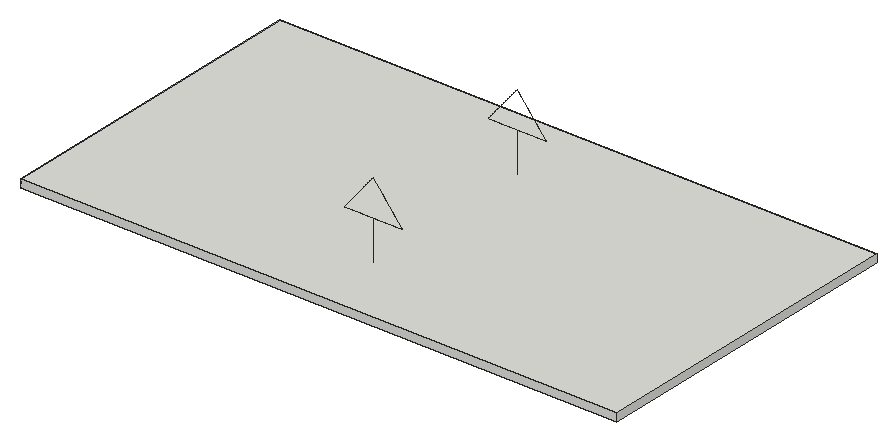
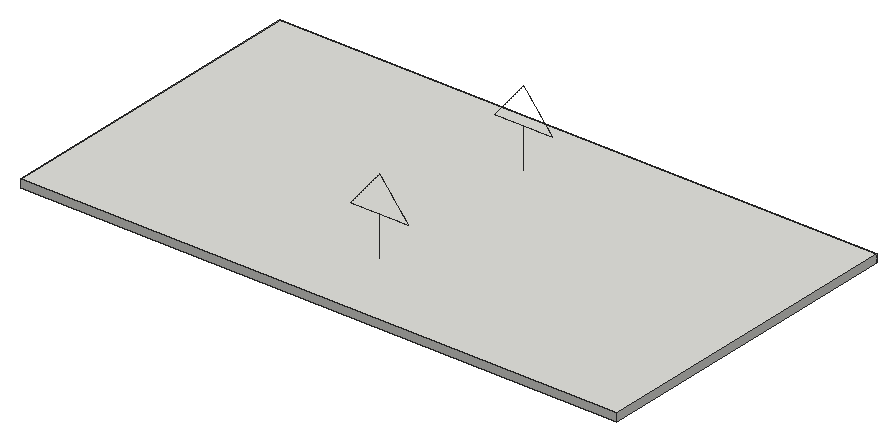
# SketchUp Ruby script. Lengths in inches.
U = 1.inch
M = Sketchup.active_model
def pt(a) = Geom::Point3d.new(a.map { |v| v * U })
def face(e, loops, mat)
  f = e.add_face(loops[0].map { |a| pt(a) })
  loops[1..].each { |l| e.add_face(l.map { |a| pt(a) }).erase! }
  f.material = f.back_material = mat if mat
  f
end
# faces: each face lists its corners as indices into pts; further lists are holes
def faces(e, pts, list, mat = nil) = list.each { |f| face(e, (f[0].is_a?(Array) ? f : [f]).map { |l| l.map { |i| pts[i] } }, mat) }
# xy, xz, yz: faces in a plane at the given z, y or x. An outline is a flat list of corners, or four numbers for a rectangle; further outlines are holes
def ring(l) = l.size == 4 ? [[l[0], l[1]], [l[2], l[1]], [l[2], l[3]], [l[0], l[3]]] : l.each_slice(2).to_a
def flat(e, list, mat, &to3) = list.each { |f| face(e, (f[0].is_a?(Array) ? f : [f]).map { |l| ring(l).map { |u, v| to3.(u, v) } }, mat) }
def xy(e, z, list, mat = nil) = flat(e, list, mat) { |x, y| [x, y, z] }
def xz(e, y, list, mat = nil) = flat(e, list, mat) { |x, z| [x, y, z] }
def yz(e, x, list, mat = nil) = flat(e, list, mat) { |y, z| [x, y, z] }
def lines(e, pts, list) = list.each { |a, b| e.add_line(pt(pts[a]), pt(pts[b])) }
# prism: a flat outline (further loops are holes) pulled along v
def prism(e, loops, v, mat = nil)
  f = face(e, loops, mat); d = Geom::Vector3d.new(v.map { |x| x * U })
  f.pushpull(f.normal.samedirection?(d) ? d.length : -d.length)
end
def box(e, o, s, mat = nil) = prism(e, [[o, [o[0] + s[0], o[1], o[2]], [o[0] + s[0], o[1] + s[1], o[2]], [o[0], o[1] + s[1], o[2]]]], [0, 0, s[2]], mat)
def at(x, y, z, deg = 0) = Geom::Transformation.translation(pt([x, y, z])) * Geom::Transformation.rotation(ORIGIN, Z_AXIS, deg.degrees)
def axes(o, x, y, z) = Geom::Transformation.new([*x, 0, *y, 0, *z, 0, *pt(o).to_a, 1])
def part(name) = M.definitions.add(name)
# library, detail: a bought-in or finely detailed component or shape, given as its bounding box
def library(name, o, s) = part(name).tap { |d| box(d.entities, o, s) }
def detail(e, o, s) = box(e.add_group.entities, o, s)
def put(e, d, t, mat = nil) = e.add_instance(d, t).tap { |i| i.material = mat if mat }
def group(e, t, mat = nil) = e.add_group.tap { |g| g.transformation = t; g.material = mat if mat }.entities
root = M.entities
c1 = part("Group84\#1")
p = [[0,0,0],[0,0,-43.36],[-21.49,0,-43.36],[139.88,-0.5,0],[-139.88,-0.5,0],[139.88,0.5,0],
  [139.88,0,0],[-139.88,0.5,0],[21.49,0,-43.36],[-139.88,0,0],[0,0,-70.19]]
lines(c1.entities,p,[[0,1],[1,2],[3,4],[5,6],[7,5],[1,8],[9,0],[0,6],[8,10],[4,9],[6,3],[2,10],
  [9,7]])
c2 = part("Rectangle Light")
put(c2.entities,c1,at(0,0,0))
c3 = part("Group")
box(c3.entities,[0,0,0],[440.75,240,6])
xy(root,232,[[[79.99,50,360.75,184],[80.99,51,359.75,183]]])
xy(root,233,[[[80.99,51,359.75,183],[81.99,52,358.75,182]]])
xy(root,234,[[[57.99,28,382.75,206],[79.99,50,360.75,184],[370.5625,111,370.19,111.03,369.8125,111.07,369.44,111.14,369.08,111.24,368.72,111.35,368.37,111.49,368.03,111.65,367.7,111.84,367.38,112.04,367.07,112.26,366.78,112.5,366.51,112.76,366.25,113.03,366.01,113.32,365.79,113.63,365.59,113.95,365.4,114.28,365.24,114.62,365.1,114.97,364.99,115.33,364.89,115.69,364.82,116.0625,364.78,116.44,364.75,116.8125,364.75,117.1875,364.78,117.56,364.82,117.9375,364.89,118.31,364.99,118.67,365.1,119.03,365.24,119.38,365.4,119.72,365.59,120.05,365.79,120.37,366.01,120.68,366.25,120.97,366.51,121.24,366.78,121.5,367.07,121.74,367.38,121.96,367.7,122.16,368.03,122.35,368.37,122.51,368.72,122.65,369.08,122.76,369.44,122.86,369.8125,122.93,370.19,122.97,370.5625,123,370.9375,123,371.31,122.97,371.6875,122.93,372.06,122.86,372.42,122.76,372.78,122.65,373.13,122.51,373.47,122.35,373.8,122.16,374.12,121.96,374.43,121.74,374.72,121.5,374.99,121.24,375.25,120.97,375.49,120.68,375.71,120.37,375.91,120.05,376.1,119.72,376.26,119.38,376.4,119.03,376.51,118.67,376.61,118.31,376.68,117.9375,376.72,117.56,376.75,117.1875,376.75,116.8125,376.72,116.44,376.68,116.0625,376.61,115.69,376.51,115.33,376.4,114.97,376.26,114.62,376.1,114.28,375.91,113.95,375.71,113.63,375.49,113.32,375.25,113.03,374.99,112.76,374.72,112.5,374.43,112.26,374.12,112.04,373.8,111.84,373.47,111.65,373.13,111.49,372.78,111.35,372.42,111.24,372.06,111.14,371.6875,111.07,371.31,111.03,370.9375,111],[220.18,34,219.81,34.03,219.43,34.07,219.0625,34.14,218.7,34.24,218.34,34.35,217.99,34.49,217.65,34.65,217.32,34.84,217,35.04,216.69,35.26,216.4,35.5,216.13,35.76,215.87,36.03,215.63,36.32,215.41,36.63,215.21,36.95,215.02,37.28,214.86,37.62,214.73,37.97,214.61,38.33,214.52,38.69,214.44,39.0625,214.4,39.44,214.375,39.8125,214.375,40.1875,214.4,40.56,214.44,40.9375,214.52,41.31,214.61,41.67,214.73,42.03,214.86,42.38,215.02,42.72,215.21,43.05,215.41,43.37,215.63,43.68,215.87,43.97,216.13,44.24,216.4,44.5,216.69,44.74,217,44.96,217.32,45.16,217.65,45.35,217.99,45.51,218.34,45.65,218.7,45.76,219.0625,45.86,219.43,45.93,219.81,45.97,220.18,46,220.56,46,220.94,45.97,221.31,45.93,221.68,45.86,222.04,45.76,222.4,45.65,222.75,45.51,223.09,45.35,223.43,45.16,223.74,44.96,224.05,44.74,224.34,44.5,224.61,44.24,224.87,43.97,225.11,43.68,225.33,43.37,225.54,43.05,225.72,42.72,225.88,42.38,226.02,42.03,226.13,41.67,226.23,41.31,226.3,40.9375,226.34,40.56,226.37,40.1875,226.37,39.8125,226.34,39.44,226.3,39.0625,226.23,38.69,226.13,38.33,226.02,37.97,225.88,37.62,225.72,37.28,225.54,36.95,225.33,36.63,225.11,36.32,224.87,36.03,224.61,35.76,224.34,35.5,224.05,35.26,223.74,35.04,223.43,34.84,223.09,34.65,222.75,34.49,222.4,34.35,222.04,34.24,221.68,34.14,221.31,34.07,220.94,34.03,220.56,34],[295.37,34,295,34.03,294.62,34.07,294.25,34.14,293.89,34.24,293.53,34.35,293.18,34.49,292.84,34.65,292.51,34.84,292.1875,35.04,291.88,35.26,291.59,35.5,291.32,35.76,291.06,36.03,290.82,36.32,290.6,36.63,290.4,36.95,290.21,37.28,290.05,37.62,289.92,37.97,289.8,38.33,289.7,38.69,289.63,39.0625,289.59,39.44,289.5625,39.8125,289.5625,40.1875,289.59,40.56,289.63,40.9375,289.7,41.31,289.8,41.67,289.92,42.03,290.05,42.38,290.21,42.72,290.4,43.05,290.6,43.37,290.82,43.68,291.06,43.97,291.32,44.24,291.59,44.5,291.88,44.74,292.1875,44.96,292.51,45.16,292.84,45.35,293.18,45.51,293.53,45.65,293.89,45.76,294.25,45.86,294.62,45.93,295,45.97,295.37,46,295.75,46,296.125,45.97,296.5,45.93,296.87,45.86,297.23,45.76,297.59,45.65,297.94,45.51,298.28,45.35,298.61,45.16,298.93,44.96,299.24,44.74,299.53,44.5,299.8,44.24,300.0625,43.97,300.3,43.68,300.52,43.37,300.72,43.05,300.91,42.72,301.07,42.38,301.21,42.03,301.32,41.67,301.42,41.31,301.49,40.9375,301.53,40.56,301.56,40.1875,301.56,39.8125,301.53,39.44,301.49,39.0625,301.42,38.69,301.32,38.33,301.21,37.97,301.07,37.62,300.91,37.28,300.72,36.95,300.52,36.63,300.3,36.32,300.0625,36.03,299.8,35.76,299.53,35.5,299.24,35.26,298.93,35.04,298.61,34.84,298.28,34.65,297.94,34.49,297.59,34.35,297.23,34.24,296.87,34.14,296.5,34.07,296.125,34.03,295.75,34],[370.5625,34,370.19,34.03,369.8125,34.07,369.44,34.14,369.08,34.24,368.72,34.35,368.37,34.49,368.03,34.65,367.7,34.84,367.38,35.04,367.07,35.26,366.78,35.5,366.51,35.76,366.25,36.03,366.01,36.32,365.79,36.63,365.59,36.95,365.4,37.28,365.24,37.62,365.1,37.97,364.99,38.33,364.89,38.69,364.82,39.0625,364.78,39.44,364.75,39.8125,364.75,40.1875,364.78,40.56,364.82,40.9375,364.89,41.31,364.99,41.67,365.1,42.03,365.24,42.38,365.4,42.72,365.59,43.05,365.79,43.37,366.01,43.68,366.25,43.97,366.51,44.24,366.78,44.5,367.07,44.74,367.38,44.96,367.7,45.16,368.03,45.35,368.37,45.51,368.72,45.65,369.08,45.76,369.44,45.86,369.8125,45.93,370.19,45.97,370.5625,46,370.9375,46,371.31,45.97,371.6875,45.93,372.06,45.86,372.42,45.76,372.78,45.65,373.13,45.51,373.47,45.35,373.8,45.16,374.12,44.96,374.43,44.74,374.72,44.5,374.99,44.24,375.25,43.97,375.49,43.68,375.71,43.37,375.91,43.05,376.1,42.72,376.26,42.38,376.4,42.03,376.51,41.67,376.61,41.31,376.68,40.9375,376.72,40.56,376.75,40.1875,376.75,39.8125,376.72,39.44,376.68,39.0625,376.61,38.69,376.51,38.33,376.4,37.97,376.26,37.62,376.1,37.28,375.91,36.95,375.71,36.63,375.49,36.32,375.25,36.03,374.99,35.76,374.72,35.5,374.43,35.26,374.12,35.04,373.8,34.84,373.47,34.65,373.13,34.49,372.78,34.35,372.42,34.24,372.06,34.14,371.6875,34.07,371.31,34.03,370.9375,34],[144.99,188,144.62,188.03,144.24,188.07,143.87,188.14,143.51,188.24,143.15,188.35,142.8,188.49,142.46,188.65,142.125,188.84,141.81,189.04,141.5,189.26,141.21,189.5,140.9375,189.76,140.68,190.03,140.44,190.32,140.22,190.63,140.02,190.95,139.84,191.28,139.67,191.62,139.54,191.97,139.42,192.33,139.33,192.69,139.26,193.0625,139.21,193.44,139.18,193.8125,139.18,194.1875,139.21,194.56,139.26,194.9375,139.33,195.31,139.42,195.67,139.54,196.03,139.67,196.38,139.84,196.72,140.02,197.05,140.22,197.37,140.44,197.68,140.68,197.97,140.9375,198.24,141.21,198.5,141.5,198.74,141.81,198.96,142.125,199.16,142.46,199.35,142.8,199.51,143.15,199.65,143.51,199.76,143.87,199.86,144.24,199.93,144.62,199.97,144.99,200,145.37,200,145.75,199.97,146.12,199.93,146.49,199.86,146.86,199.76,147.21,199.65,147.5625,199.51,147.91,199.35,148.24,199.16,148.55,198.96,148.86,198.74,149.15,198.5,149.42,198.24,149.68,197.97,149.92,197.68,150.14,197.37,150.35,197.05,150.53,196.72,150.6875,196.38,150.83,196.03,150.94,195.67,151.04,195.31,151.11,194.9375,151.15,194.56,151.18,194.1875,151.18,193.8125,151.15,193.44,151.11,193.0625,151.04,192.69,150.94,192.33,150.83,191.97,150.6875,191.62,150.53,191.28,150.35,190.95,150.14,190.63,149.92,190.32,149.68,190.03,149.42,189.76,149.15,189.5,148.86,189.26,148.55,189.04,148.24,188.84,147.91,188.65,147.5625,188.49,147.21,188.35,146.86,188.24,146.49,188.14,146.12,188.07,145.75,188.03,145.37,188],[69.8,188,69.43,188.03,69.05,188.07,68.68,188.14,68.32,188.24,67.96,188.35,67.61,188.49,67.27,188.65,66.9375,188.84,66.62,189.04,66.3125,189.26,66.02,189.5,65.75,189.76,65.49,190.03,65.25,190.32,65.03,190.63,64.83,190.95,64.65,191.28,64.48,191.62,64.35,191.97,64.23,192.33,64.14,192.69,64.07,193.0625,64.02,193.44,63.99,193.8125,63.99,194.1875,64.02,194.56,64.07,194.9375,64.14,195.31,64.23,195.67,64.35,196.03,64.48,196.38,64.65,196.72,64.83,197.05,65.03,197.37,65.25,197.68,65.49,197.97,65.75,198.24,66.02,198.5,66.3125,198.74,66.62,198.96,66.9375,199.16,67.27,199.35,67.61,199.51,67.96,199.65,68.32,199.76,68.68,199.86,69.05,199.93,69.43,199.97,69.8,200,70.18,200,70.56,199.97,70.93,199.93,71.3,199.86,71.67,199.76,72.02,199.65,72.375,199.51,72.72,199.35,73.05,199.16,73.36,198.96,73.67,198.74,73.96,198.5,74.23,198.24,74.49,197.97,74.73,197.68,74.95,197.37,75.16,197.05,75.34,196.72,75.5,196.38,75.64,196.03,75.75,195.67,75.85,195.31,75.92,194.9375,75.96,194.56,75.99,194.1875,75.99,193.8125,75.96,193.44,75.92,193.0625,75.85,192.69,75.75,192.33,75.64,191.97,75.5,191.62,75.34,191.28,75.16,190.95,74.95,190.63,74.73,190.32,74.49,190.03,74.23,189.76,73.96,189.5,73.67,189.26,73.36,189.04,73.05,188.84,72.72,188.65,72.375,188.49,72.02,188.35,71.67,188.24,71.3,188.14,70.93,188.07,70.56,188.03,70.18,188],[69.8,111,69.43,111.03,69.05,111.07,68.68,111.14,68.32,111.24,67.96,111.35,67.61,111.49,67.27,111.65,66.9375,111.84,66.62,112.04,66.3125,112.26,66.02,112.5,65.75,112.76,65.49,113.03,65.25,113.32,65.03,113.63,64.83,113.95,64.65,114.28,64.48,114.62,64.35,114.97,64.23,115.33,64.14,115.69,64.07,116.0625,64.02,116.44,63.99,116.8125,63.99,117.1875,64.02,117.56,64.07,117.9375,64.14,118.31,64.23,118.67,64.35,119.03,64.48,119.38,64.65,119.72,64.83,120.05,65.03,120.37,65.25,120.68,65.49,120.97,65.75,121.24,66.02,121.5,66.3125,121.74,66.62,121.96,66.9375,122.16,67.27,122.35,67.61,122.51,67.96,122.65,68.32,122.76,68.68,122.86,69.05,122.93,69.43,122.97,69.8,123,70.18,123,70.56,122.97,70.93,122.93,71.3,122.86,71.67,122.76,72.02,122.65,72.375,122.51,72.72,122.35,73.05,122.16,73.36,121.96,73.67,121.74,73.96,121.5,74.23,121.24,74.49,120.97,74.73,120.68,74.95,120.37,75.16,120.05,75.34,119.72,75.5,119.38,75.64,119.03,75.75,118.67,75.85,118.31,75.92,117.9375,75.96,117.56,75.99,117.1875,75.99,116.8125,75.96,116.44,75.92,116.0625,75.85,115.69,75.75,115.33,75.64,114.97,75.5,114.62,75.34,114.28,75.16,113.95,74.95,113.63,74.73,113.32,74.49,113.03,74.23,112.76,73.96,112.5,73.67,112.26,73.36,112.04,73.05,111.84,72.72,111.65,72.375,111.49,72.02,111.35,71.67,111.24,71.3,111.14,70.93,111.07,70.56,111.03,70.18,111],[370.5625,188,370.19,188.03,369.8125,188.07,369.44,188.14,369.08,188.24,368.72,188.35,368.37,188.49,368.03,188.65,367.7,188.84,367.38,189.04,367.07,189.26,366.78,189.5,366.51,189.76,366.25,190.03,366.01,190.32,365.79,190.63,365.59,190.95,365.4,191.28,365.24,191.62,365.1,191.97,364.99,192.33,364.89,192.69,364.82,193.0625,364.78,193.44,364.75,193.8125,364.75,194.1875,364.78,194.56,364.82,194.9375,364.89,195.31,364.99,195.67,365.1,196.03,365.24,196.38,365.4,196.72,365.59,197.05,365.79,197.37,366.01,197.68,366.25,197.97,366.51,198.24,366.78,198.5,367.07,198.74,367.38,198.96,367.7,199.16,368.03,199.35,368.37,199.51,368.72,199.65,369.08,199.76,369.44,199.86,369.8125,199.93,370.19,199.97,370.5625,200,370.9375,200,371.31,199.97,371.6875,199.93,372.06,199.86,372.42,199.76,372.78,199.65,373.13,199.51,373.47,199.35,373.8,199.16,374.12,198.96,374.43,198.74,374.72,198.5,374.99,198.24,375.25,197.97,375.49,197.68,375.71,197.37,375.91,197.05,376.1,196.72,376.26,196.38,376.4,196.03,376.51,195.67,376.61,195.31,376.68,194.9375,376.72,194.56,376.75,194.1875,376.75,193.8125,376.72,193.44,376.68,193.0625,376.61,192.69,376.51,192.33,376.4,191.97,376.26,191.62,376.1,191.28,375.91,190.95,375.71,190.63,375.49,190.32,375.25,190.03,374.99,189.76,374.72,189.5,374.43,189.26,374.12,189.04,373.8,188.84,373.47,188.65,373.13,188.49,372.78,188.35,372.42,188.24,372.06,188.14,371.6875,188.07,371.31,188.03,370.9375,188],[295.37,188,295,188.03,294.62,188.07,294.25,188.14,293.89,188.24,293.53,188.35,293.18,188.49,292.84,188.65,292.51,188.84,292.1875,189.04,291.88,189.26,291.59,189.5,291.32,189.76,291.06,190.03,290.82,190.32,290.6,190.63,290.4,190.95,290.21,191.28,290.05,191.62,289.92,191.97,289.8,192.33,289.7,192.69,289.63,193.0625,289.59,193.44,289.5625,193.8125,289.5625,194.1875,289.59,194.56,289.63,194.9375,289.7,195.31,289.8,195.67,289.92,196.03,290.05,196.38,290.21,196.72,290.4,197.05,290.6,197.37,290.82,197.68,291.06,197.97,291.32,198.24,291.59,198.5,291.88,198.74,292.1875,198.96,292.51,199.16,292.84,199.35,293.18,199.51,293.53,199.65,293.89,199.76,294.25,199.86,294.62,199.93,295,199.97,295.37,200,295.75,200,296.125,199.97,296.5,199.93,296.87,199.86,297.23,199.76,297.59,199.65,297.94,199.51,298.28,199.35,298.61,199.16,298.93,198.96,299.24,198.74,299.53,198.5,299.8,198.24,300.0625,197.97,300.3,197.68,300.52,197.37,300.72,197.05,300.91,196.72,301.07,196.38,301.21,196.03,301.32,195.67,301.42,195.31,301.49,194.9375,301.53,194.56,301.56,194.1875,301.56,193.8125,301.53,193.44,301.49,193.0625,301.42,192.69,301.32,192.33,301.21,191.97,301.07,191.62,300.91,191.28,300.72,190.95,300.52,190.63,300.3,190.32,300.0625,190.03,299.8,189.76,299.53,189.5,299.24,189.26,298.93,189.04,298.61,188.84,298.28,188.65,297.94,188.49,297.59,188.35,297.23,188.24,296.87,188.14,296.5,188.07,296.125,188.03,295.75,188],[220.18,188,219.81,188.03,219.43,188.07,219.0625,188.14,218.7,188.24,218.34,188.35,217.99,188.49,217.65,188.65,217.32,188.84,217,189.04,216.69,189.26,216.4,189.5,216.13,189.76,215.87,190.03,215.63,190.32,215.41,190.63,215.21,190.95,215.02,191.28,214.86,191.62,214.73,191.97,214.61,192.33,214.52,192.69,214.44,193.0625,214.4,193.44,214.375,193.8125,214.375,194.1875,214.4,194.56,214.44,194.9375,214.52,195.31,214.61,195.67,214.73,196.03,214.86,196.38,215.02,196.72,215.21,197.05,215.41,197.37,215.63,197.68,215.87,197.97,216.13,198.24,216.4,198.5,216.69,198.74,217,198.96,217.32,199.16,217.65,199.35,217.99,199.51,218.34,199.65,218.7,199.76,219.0625,199.86,219.43,199.93,219.81,199.97,220.18,200,220.56,200,220.94,199.97,221.31,199.93,221.68,199.86,222.04,199.76,222.4,199.65,222.75,199.51,223.09,199.35,223.43,199.16,223.74,198.96,224.05,198.74,224.34,198.5,224.61,198.24,224.87,197.97,225.11,197.68,225.33,197.37,225.54,197.05,225.72,196.72,225.88,196.38,226.02,196.03,226.13,195.67,226.23,195.31,226.3,194.9375,226.34,194.56,226.37,194.1875,226.37,193.8125,226.34,193.44,226.3,193.0625,226.23,192.69,226.13,192.33,226.02,191.97,225.88,191.62,225.72,191.28,225.54,190.95,225.33,190.63,225.11,190.32,224.87,190.03,224.61,189.76,224.34,189.5,224.05,189.26,223.74,189.04,223.43,188.84,223.09,188.65,222.75,188.49,222.4,188.35,222.04,188.24,221.68,188.14,221.31,188.07,220.94,188.03,220.56,188],[69.8,34,69.43,34.03,69.05,34.07,68.68,34.14,68.32,34.24,67.96,34.35,67.61,34.49,67.27,34.65,66.9375,34.84,66.62,35.04,66.3125,35.26,66.02,35.5,65.75,35.76,65.49,36.03,65.25,36.32,65.03,36.63,64.83,36.95,64.65,37.28,64.48,37.62,64.35,37.97,64.23,38.33,64.14,38.69,64.07,39.0625,64.02,39.44,63.99,39.8125,63.99,40.1875,64.02,40.56,64.07,40.9375,64.14,41.31,64.23,41.67,64.35,42.03,64.48,42.38,64.65,42.72,64.83,43.05,65.03,43.37,65.25,43.68,65.49,43.97,65.75,44.24,66.02,44.5,66.3125,44.74,66.62,44.96,66.9375,45.16,67.27,45.35,67.61,45.51,67.96,45.65,68.32,45.76,68.68,45.86,69.05,45.93,69.43,45.97,69.8,46,70.18,46,70.56,45.97,70.93,45.93,71.3,45.86,71.67,45.76,72.02,45.65,72.375,45.51,72.72,45.35,73.05,45.16,73.36,44.96,73.67,44.74,73.96,44.5,74.23,44.24,74.49,43.97,74.73,43.68,74.95,43.37,75.16,43.05,75.34,42.72,75.5,42.38,75.64,42.03,75.75,41.67,75.85,41.31,75.92,40.9375,75.96,40.56,75.99,40.1875,75.99,39.8125,75.96,39.44,75.92,39.0625,75.85,38.69,75.75,38.33,75.64,37.97,75.5,37.62,75.34,37.28,75.16,36.95,74.95,36.63,74.73,36.32,74.49,36.03,74.23,35.76,73.96,35.5,73.67,35.26,73.36,35.04,73.05,34.84,72.72,34.65,72.375,34.49,72.02,34.35,71.67,34.24,71.3,34.14,70.93,34.07,70.56,34.03,70.18,34],[144.99,34,144.62,34.03,144.24,34.07,143.87,34.14,143.51,34.24,143.15,34.35,142.8,34.49,142.46,34.65,142.125,34.84,141.81,35.04,141.5,35.26,141.21,35.5,140.9375,35.76,140.68,36.03,140.44,36.32,140.22,36.63,140.02,36.95,139.84,37.28,139.67,37.62,139.54,37.97,139.42,38.33,139.33,38.69,139.26,39.0625,139.21,39.44,139.18,39.8125,139.18,40.1875,139.21,40.56,139.26,40.9375,139.33,41.31,139.42,41.67,139.54,42.03,139.67,42.38,139.84,42.72,140.02,43.05,140.22,43.37,140.44,43.68,140.68,43.97,140.9375,44.24,141.21,44.5,141.5,44.74,141.81,44.96,142.125,45.16,142.46,45.35,142.8,45.51,143.15,45.65,143.51,45.76,143.87,45.86,144.24,45.93,144.62,45.97,144.99,46,145.37,46,145.75,45.97,146.12,45.93,146.49,45.86,146.86,45.76,147.21,45.65,147.5625,45.51,147.91,45.35,148.24,45.16,148.55,44.96,148.86,44.74,149.15,44.5,149.42,44.24,149.68,43.97,149.92,43.68,150.14,43.37,150.35,43.05,150.53,42.72,150.6875,42.38,150.83,42.03,150.94,41.67,151.04,41.31,151.11,40.9375,151.15,40.56,151.18,40.1875,151.18,39.8125,151.15,39.44,151.11,39.0625,151.04,38.69,150.94,38.33,150.83,37.97,150.6875,37.62,150.53,37.28,150.35,36.95,150.14,36.63,149.92,36.32,149.68,36.03,149.42,35.76,149.15,35.5,148.86,35.26,148.55,35.04,148.24,34.84,147.91,34.65,147.5625,34.49,147.21,34.35,146.86,34.24,146.49,34.14,146.12,34.07,145.75,34.03,145.37,34]],[79.99,50,360.75,184]])
xz(root,50,[[79.99,232,360.75,234]])
xz(root,51,[[80.99,232,359.75,233]])
xz(root,183,[[80.99,232,359.75,233]])
xz(root,184,[[79.99,232,360.75,234]])
xz(root,188,[[144.99,231.53,145.37,234],[220.18,231.53,220.56,234]])
xz(root,200,[[144.99,231.53,145.37,234],[220.18,231.53,220.56,234]])
yz(root,151.18,[[193.8125,231.53,194.1875,234]])
yz(root,214.375,[[193.8125,231.53,194.1875,234]])
p = [[144.62,188.03,231.53],[144.24,188.07,231.53],[144.24,188.07,234],[144.62,188.03,234],[144.99,188,231.53],[144.99,188,234],
  [145.75,188.03,231.53],[145.37,188,231.53],[145.37,188,234],[145.75,188.03,234],[146.12,188.07,231.53],[146.12,188.07,234],
  [219.81,188.03,231.53],[219.43,188.07,231.53],[219.43,188.07,234],[219.81,188.03,234],[220.18,188,231.53],[220.18,188,234],
  [220.94,188.03,231.53],[220.56,188,231.53],[220.56,188,234],[220.94,188.03,234],[221.31,188.07,231.53],[221.31,188.07,234],
  [143.87,188.14,231.53],[143.51,188.24,231.53],[143.51,188.24,234],[143.87,188.14,234],[146.49,188.14,231.53],[146.49,188.14,234],
  [146.86,188.24,231.53],[146.86,188.24,234],[219.0625,188.14,231.53],[218.7,188.24,231.53],[218.7,188.24,234],[219.0625,188.14,234],
  [143.15,188.35,231.53],[143.15,188.35,234],[147.21,188.35,231.53],[147.21,188.35,234],[218.34,188.35,231.53],[218.34,188.35,234],
  [142.8,188.49,231.53],[142.8,188.49,234],[147.5625,188.49,231.53],[147.5625,188.49,234],[217.99,188.49,231.53],[217.99,188.49,234],
  [142.46,188.65,231.53],[142.46,188.65,234],[147.91,188.65,231.53],[147.91,188.65,234],[217.65,188.65,231.53],[217.65,188.65,234],
  [142.125,188.84,231.53],[142.125,188.84,234],[148.24,188.84,231.53],[148.24,188.84,234],[217.32,188.84,231.53],[217.32,188.84,234],
  [141.81,189.04,231.53],[141.81,189.04,234],[148.55,189.04,231.53],[148.55,189.04,234],[217,189.04,231.53],[217,189.04,234],
  [141.5,189.26,231.53],[141.5,189.26,234],[148.86,189.26,231.53],[148.86,189.26,234],[216.69,189.26,231.53],[216.69,189.26,234],
  [141.21,189.5,231.53],[141.21,189.5,234],[149.15,189.5,231.53],[149.15,189.5,234],[216.4,189.5,231.53],[216.4,189.5,234],
  [140.9375,189.76,231.53],[140.9375,189.76,234],[149.42,189.76,231.53],[149.42,189.76,234],[216.13,189.76,231.53],[216.13,189.76,234],
  [140.68,190.03,231.53],[140.68,190.03,234],[149.68,190.03,231.53],[149.68,190.03,234],[215.87,190.03,231.53],[215.87,190.03,234],
  [140.44,190.32,231.53],[140.44,190.32,234],[149.92,190.32,231.53],[149.92,190.32,234],[215.63,190.32,231.53],[215.63,190.32,234],
  [140.22,190.63,231.53],[140.22,190.63,234],[150.14,190.63,231.53],[150.14,190.63,234],[215.41,190.63,231.53],[215.41,190.63,234],
  [140.02,190.95,231.53],[140.02,190.95,234],[150.35,190.95,231.53],[150.35,190.95,234],[215.21,190.95,231.53],[215.21,190.95,234],
  [139.84,191.28,231.53],[139.84,191.28,234],[150.53,191.28,231.53],[150.53,191.28,234],[215.02,191.28,231.53],[215.02,191.28,234],
  [139.67,191.62,231.53],[139.67,191.62,234],[150.6875,191.62,231.53],[150.6875,191.62,234],[214.86,191.62,231.53],[214.86,191.62,234],
  [139.54,191.97,231.53],[139.54,191.97,234],[150.83,191.97,231.53],[150.83,191.97,234],[214.73,191.97,231.53],[214.73,191.97,234],
  [139.42,192.33,231.53],[139.42,192.33,234],[150.94,192.33,231.53],[150.94,192.33,234],[214.61,192.33,231.53],[214.61,192.33,234],
  [151.04,192.69,231.53],[151.04,192.69,234],[214.52,192.69,231.53],[214.52,192.69,234],[151.11,193.0625,231.53],[151.11,193.0625,234],
  [214.44,193.0625,231.53],[214.44,193.0625,234],[151.15,193.44,231.53],[151.15,193.44,234],[214.4,193.44,231.53],[214.4,193.44,234],
  [151.18,193.8125,231.53],[151.18,193.8125,234],[214.375,193.8125,231.53],[214.375,193.8125,234],[151.15,194.56,231.53],[151.18,194.1875,231.53],
  [151.18,194.1875,234],[151.15,194.56,234],[214.375,194.1875,231.53],[214.4,194.56,231.53],[214.4,194.56,234],[214.375,194.1875,234],
  [151.11,194.9375,231.53],[151.11,194.9375,234],[214.44,194.9375,231.53],[214.44,194.9375,234],[151.04,195.31,231.53],[151.04,195.31,234],
  [214.52,195.31,231.53],[214.52,195.31,234],[150.94,195.67,231.53],[150.94,195.67,234],[214.61,195.67,231.53],[214.61,195.67,234],
  [139.42,195.67,231.53],[139.54,196.03,231.53],[139.54,196.03,234],[139.42,195.67,234],[150.83,196.03,231.53],[150.83,196.03,234],
  [214.73,196.03,231.53],[214.73,196.03,234],[139.67,196.38,231.53],[139.67,196.38,234],[150.6875,196.38,231.53],[150.6875,196.38,234],
  [214.86,196.38,231.53],[214.86,196.38,234],[139.84,196.72,231.53],[139.84,196.72,234],[150.53,196.72,231.53],[150.53,196.72,234],
  [215.02,196.72,231.53],[215.02,196.72,234],[140.02,197.05,231.53],[140.02,197.05,234],[150.35,197.05,231.53],[150.35,197.05,234],
  [215.21,197.05,231.53],[215.21,197.05,234],[140.22,197.37,231.53],[140.22,197.37,234],[150.14,197.37,231.53],[150.14,197.37,234],
  [215.41,197.37,231.53],[215.41,197.37,234],[140.44,197.68,231.53],[140.44,197.68,234],[149.92,197.68,231.53],[149.92,197.68,234],
  [215.63,197.68,231.53],[215.63,197.68,234],[140.68,197.97,231.53],[140.68,197.97,234],[149.68,197.97,231.53],[149.68,197.97,234],
  [215.87,197.97,231.53],[215.87,197.97,234],[140.9375,198.24,231.53],[140.9375,198.24,234],[149.42,198.24,231.53],[149.42,198.24,234],
  [216.13,198.24,231.53],[216.13,198.24,234],[141.21,198.5,231.53],[141.21,198.5,234],[149.15,198.5,231.53],[149.15,198.5,234],
  [216.4,198.5,231.53],[216.4,198.5,234],[141.5,198.74,231.53],[141.5,198.74,234],[148.86,198.74,231.53],[148.86,198.74,234],
  [216.69,198.74,231.53],[216.69,198.74,234],[141.81,198.96,231.53],[141.81,198.96,234],[148.55,198.96,231.53],[148.55,198.96,234],
  [217,198.96,231.53],[217,198.96,234],[142.125,199.16,231.53],[142.125,199.16,234],[148.24,199.16,231.53],[148.24,199.16,234],
  [217.32,199.16,231.53],[217.32,199.16,234],[142.46,199.35,231.53],[142.46,199.35,234],[147.91,199.35,231.53],[147.91,199.35,234],
  [217.65,199.35,231.53],[217.65,199.35,234],[142.8,199.51,231.53],[142.8,199.51,234],[147.5625,199.51,231.53],[147.5625,199.51,234],
  [217.99,199.51,231.53],[217.99,199.51,234],[143.15,199.65,231.53],[143.15,199.65,234],[147.21,199.65,231.53],[147.21,199.65,234],
  [218.34,199.65,231.53],[218.34,199.65,234],[143.51,199.76,231.53],[143.51,199.76,234],[146.86,199.76,231.53],[146.86,199.76,234],
  [218.7,199.76,231.53],[218.7,199.76,234],[143.87,199.86,231.53],[143.87,199.86,234],[146.49,199.86,231.53],[146.49,199.86,234],
  [219.0625,199.86,231.53],[219.0625,199.86,234],[144.24,199.93,231.53],[144.24,199.93,234],[144.62,199.97,231.53],[144.62,199.97,234],
  [145.75,199.97,231.53],[146.12,199.93,231.53],[146.12,199.93,234],[145.75,199.97,234],[219.43,199.93,231.53],[219.43,199.93,234],
  [219.81,199.97,231.53],[219.81,199.97,234],[144.99,200,231.53],[144.99,200,234],[145.37,200,231.53],[145.37,200,234],
  [220.18,200,231.53],[220.18,200,234],[220.56,200,231.53],[220.94,199.97,231.53],[220.94,199.97,234],[220.56,200,234]]
faces(root,p,[[0,1,2,3],[4,0,3,5],[6,7,8,9],[10,6,9,11],[12,13,14,15],[16,12,15,17],[18,19,20,21],[22,18,21,23],
  [24,25,26,27],[1,24,27,2],[28,10,11,29],[30,28,29,31],[32,33,34,35],[13,32,35,14],[25,36,37,26],[38,30,31,39],
  [33,40,41,34],[36,42,43,37],[44,38,39,45],[40,46,47,41],[42,48,49,43],[50,44,45,51],[46,52,53,47],[48,54,55,49],
  [56,50,51,57],[52,58,59,53],[54,60,61,55],[62,56,57,63],[58,64,65,59],[60,66,67,61],[68,62,63,69],[64,70,71,65],
  [66,72,73,67],[74,68,69,75],[70,76,77,71],[72,78,79,73],[80,74,75,81],[76,82,83,77],[78,84,85,79],[86,80,81,87],
  [82,88,89,83],[84,90,91,85],[92,86,87,93],[88,94,95,89],[90,96,97,91],[98,92,93,99],[94,100,101,95],[96,102,103,97],
  [104,98,99,105],[100,106,107,101],[102,108,109,103],[110,104,105,111],[106,112,113,107],[108,114,115,109],[116,110,111,117],[112,118,119,113],
  [114,120,121,115],[122,116,117,123],[118,124,125,119],[120,126,127,121],[128,122,123,129],[124,130,131,125],[132,128,129,133],[130,134,135,131],
  [136,132,133,137],[134,138,139,135],[140,136,137,141],[138,142,143,139],[144,140,141,145],[142,146,147,143],[148,149,150,151],[152,153,154,155],
  [156,148,151,157],[153,158,159,154],[160,156,157,161],[158,162,163,159],[164,160,161,165],[162,166,167,163],[168,169,170,171],[172,164,165,173],
  [166,174,175,167],[169,176,177,170],[178,172,173,179],[174,180,181,175],[176,182,183,177],[184,178,179,185],[180,186,187,181],[182,188,189,183],
  [190,184,185,191],[186,192,193,187],[188,194,195,189],[196,190,191,197],[192,198,199,193],[194,200,201,195],[202,196,197,203],[198,204,205,199],
  [200,206,207,201],[208,202,203,209],[204,210,211,205],[206,212,213,207],[214,208,209,215],[210,216,217,211],[212,218,219,213],[220,214,215,221],
  [216,222,223,217],[218,224,225,219],[226,220,221,227],[222,228,229,223],[224,230,231,225],[232,226,227,233],[228,234,235,229],[230,236,237,231],
  [238,232,233,239],[234,240,241,235],[236,242,243,237],[244,238,239,245],[240,246,247,241],[242,248,249,243],[250,244,245,251],[246,252,253,247],
  [248,254,255,249],[256,250,251,257],[252,258,259,253],[254,260,261,255],[262,256,257,263],[258,264,265,259],[260,266,267,261],[268,262,263,269],
  [264,270,271,265],[266,272,273,267],[272,274,275,273],[276,277,278,279],[277,268,269,278],[270,280,281,271],[280,282,283,281],[274,284,285,275],
  [286,276,279,287],[282,288,289,283],[290,291,292,293]])
put(root,c2,axes([220.37,183.5,232.01],[1.00357,0,0],[0,-1,0],[0,0,-1]))
put(root,c2,axes([220.37,50.5,232.01],[1.00357,0,0],[0,-1,0],[0,0,-1]))
put(root,c3,at(0,0,240))
